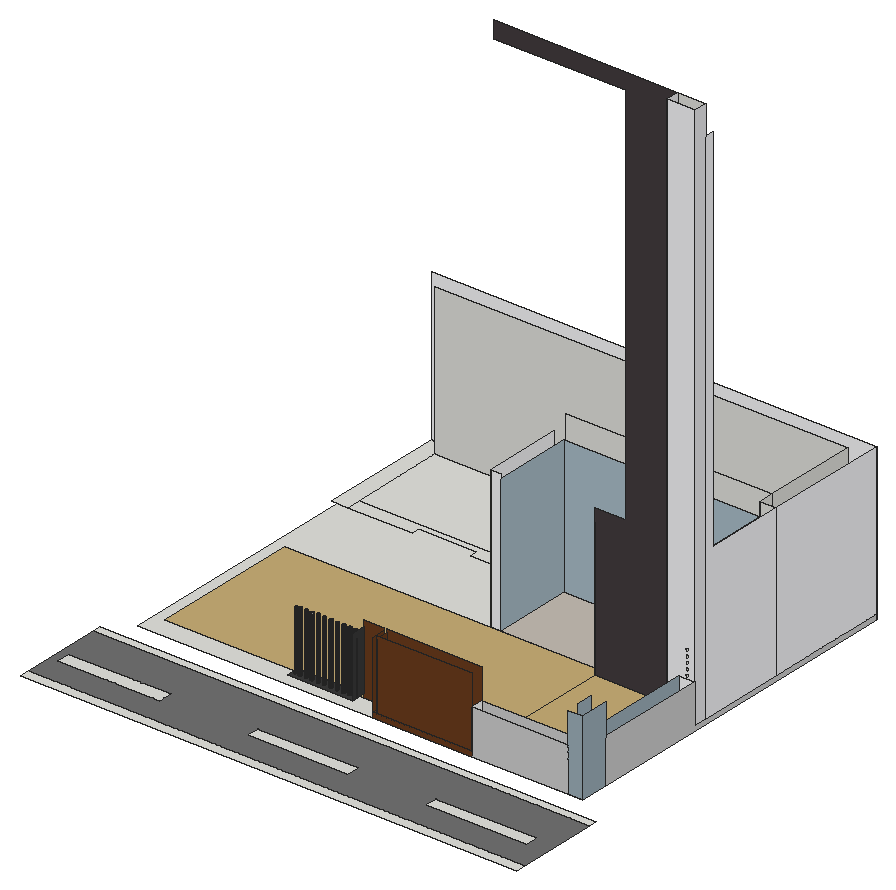
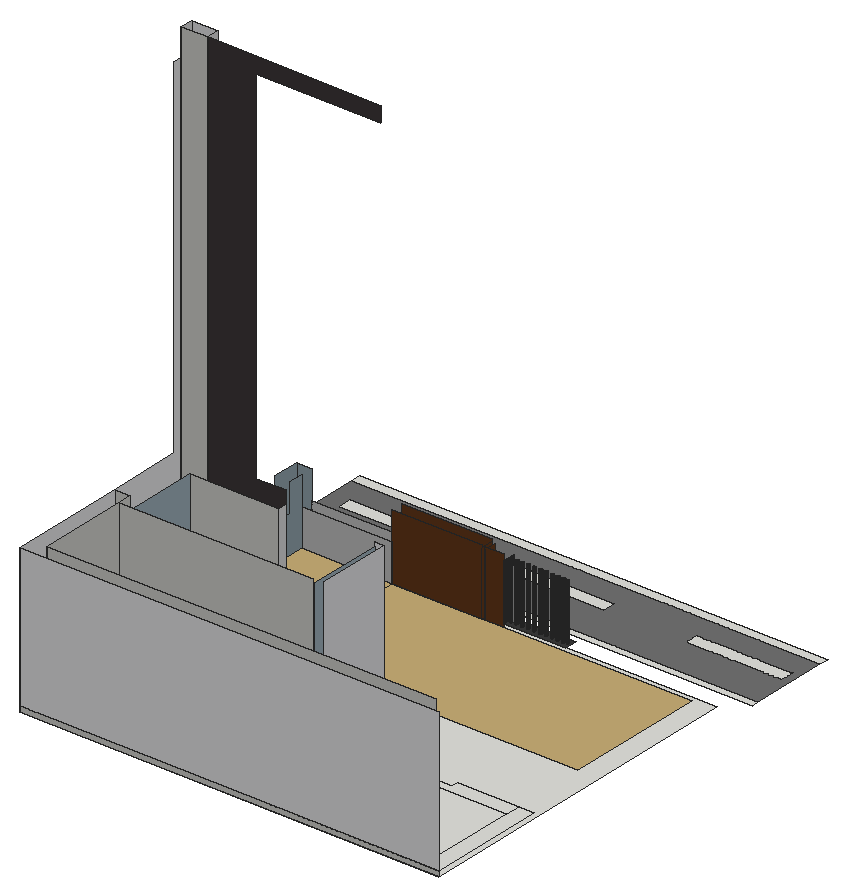
# SketchUp Ruby script. Lengths in inches.
U = 1.inch
M = Sketchup.active_model
def pt(a) = Geom::Point3d.new(a.map { |v| v * U })
def face(e, loops, mat)
  f = e.add_face(loops[0].map { |a| pt(a) })
  loops[1..].each { |l| e.add_face(l.map { |a| pt(a) }).erase! }
  f.material = f.back_material = mat if mat
  f
end
# faces: each face lists its corners as indices into pts; further lists are holes
def faces(e, pts, list, mat = nil) = list.each { |f| face(e, (f[0].is_a?(Array) ? f : [f]).map { |l| l.map { |i| pts[i] } }, mat) }
# xy, xz, yz: faces in a plane at the given z, y or x. An outline is a flat list of corners, or four numbers for a rectangle; further outlines are holes
def ring(l) = l.size == 4 ? [[l[0], l[1]], [l[2], l[1]], [l[2], l[3]], [l[0], l[3]]] : l.each_slice(2).to_a
def flat(e, list, mat, &to3) = list.each { |f| face(e, (f[0].is_a?(Array) ? f : [f]).map { |l| ring(l).map { |u, v| to3.(u, v) } }, mat) }
def xy(e, z, list, mat = nil) = flat(e, list, mat) { |x, y| [x, y, z] }
def xz(e, y, list, mat = nil) = flat(e, list, mat) { |x, z| [x, y, z] }
def yz(e, x, list, mat = nil) = flat(e, list, mat) { |y, z| [x, y, z] }
def lines(e, pts, list) = list.each { |a, b| e.add_line(pt(pts[a]), pt(pts[b])) }
# prism: a flat outline (further loops are holes) pulled along v
def prism(e, loops, v, mat = nil)
  f = face(e, loops, mat); d = Geom::Vector3d.new(v.map { |x| x * U })
  f.pushpull(f.normal.samedirection?(d) ? d.length : -d.length)
end
def box(e, o, s, mat = nil) = prism(e, [[o, [o[0] + s[0], o[1], o[2]], [o[0] + s[0], o[1] + s[1], o[2]], [o[0], o[1] + s[1], o[2]]]], [0, 0, s[2]], mat)
def at(x, y, z, deg = 0) = Geom::Transformation.translation(pt([x, y, z])) * Geom::Transformation.rotation(ORIGIN, Z_AXIS, deg.degrees)
def axes(o, x, y, z) = Geom::Transformation.new([*x, 0, *y, 0, *z, 0, *pt(o).to_a, 1])
def part(name) = M.definitions.add(name)
# library, detail: a bought-in or finely detailed component or shape, given as its bounding box
def library(name, o, s) = part(name).tap { |d| box(d.entities, o, s) }
def detail(e, o, s) = box(e.add_group.entities, o, s)
def put(e, d, t, mat = nil) = e.add_instance(d, t).tap { |i| i.material = mat if mat }
def group(e, t, mat = nil) = e.add_group.tap { |g| g.transformation = t; g.material = mat if mat }.entities
root = M.entities
M.materials.add("[Asphalt New]").color = [67, 60, 62]
M.materials.add("[Blinds Vertical Pattern]").color = [245, 245, 247]
M.materials.add("[Blinds Vertical Pattern]2").color = [234, 234, 237]
M.materials.add("[Blinds Vertical Pattern]3").color = [247, 247, 249]
M.materials.add("[Carrera Marble]").color = [207, 207, 207]
M.materials.add("[Color M03]").color = [170, 170, 170]
M.materials.add("[Color M05]").color = [114, 114, 114]
M.materials.add("[Color M07]").color = [58, 58, 58]
M.materials.add("[Field Rectangle Tile]").color = [196, 189, 179]
M.materials.add("[Formica Speckled Grey]").color = [157, 176, 186]
M.materials.add("[Formica Speckled Grey]2").color = [170, 190, 201]
M.materials.add("[Quartz Light Grey]").color = [251, 251, 252]
M.materials.add("[Tile Limestone Multi]").color = [199, 173, 118]
M.materials.add("[Wood Cherry Original]").color = [107, 60, 29]
xy(root,0,[[0,0,810.125,16.9],[13.43,59.66,179.43,82.41],[321.62,59.66,487.62,82.41],[612.68,59.66,778.68,82.41],[0,150.46,810.125,162.5625],
  [36.42,195.25,761.74,794.75]])
xy(root,0,[[[0,16.9,810.125,150.46],[13.43,59.66,179.43,82.41],[321.62,59.66,487.62,82.41],[612.68,59.66,778.68,82.41]]],"[Color M05]")
xy(root,9,[[425.33,195.25,580.71,216.53],[715.96,423.625,761.74,446.5625],[580.71,446.5625,580.71,461.03,735.46,461.03,735.46,590.55,761.74,590.55,761.74,446.5625],[399.08,461.03,399.08,590.55,262.6,590.55,262.6,602.92,168.16,602.92,168.16,590.55,62.71,590.55,62.71,614.75,735.46,614.75,735.46,590.55,415.32,590.55,415.32,461.03],[36.42,590.55,36.42,794.75,761.74,794.75,761.74,590.55,735.46,590.55,735.46,768.47,62.71,768.47,62.71,590.55],
  [62.71,614.75,735.46,768.47]])
xy(root,9,[[415.32,461.03,735.46,590.55]],"[Field Rectangle Tile]")
xy(root,9,[[62.71,216.53,580.71,461.03],[580.71,216.53,580.71,446.5625,715.96,446.5625,715.96,423.625,736.96,423.625,736.96,216.53]],"[Tile Limestone Multi]")
xy(root,9,[[420.08,195.25,425.33,216.53]],"[Wood Cherry Original]")
xy(root,14.25,[[292.65,202.87,292.05,202.95,291.49,203.18,291.01,203.55,290.64,204.03,290.41,204.58,290.33,205.18,290.41,205.78,290.64,206.34,291.01,206.82,291.49,207.18,292.05,207.42,292.65,207.49,293.24,207.42,293.8,207.18,294.28,206.82,294.65,206.34,294.88,205.78,294.96,205.18,294.88,204.58,294.65,204.03,294.28,203.55,293.8,203.18,293.24,202.95],[302.65,202.87,302.05,202.95,301.49,203.18,301.01,203.55,300.64,204.03,300.41,204.58,300.33,205.18,300.41,205.78,300.64,206.34,301.01,206.82,301.49,207.18,302.05,207.42,302.65,207.49,303.24,207.42,303.8,207.18,304.28,206.82,304.65,206.34,304.88,205.78,304.96,205.18,304.88,204.58,304.65,204.03,304.28,203.55,303.8,203.18,303.24,202.95],[312.15,202.87,311.55,202.95,310.99,203.18,310.51,203.55,310.14,204.03,309.91,204.58,309.83,205.18,309.91,205.78,310.14,206.34,310.51,206.82,310.99,207.18,311.55,207.42,312.15,207.49,312.74,207.42,313.3,207.18,313.78,206.82,314.15,206.34,314.38,205.78,314.46,205.18,314.38,204.58,314.15,204.03,313.78,203.55,313.3,203.18,312.74,202.95],[322.33,202.87,321.73,202.95,321.18,203.18,320.7,203.55,320.33,204.03,320.1,204.58,320.02,205.18,320.1,205.78,320.33,206.34,320.7,206.82,321.18,207.18,321.73,207.42,322.33,207.49,322.93,207.42,323.49,207.18,323.97,206.82,324.34,206.34,324.57,205.78,324.65,205.18,324.57,204.58,324.34,204.03,323.97,203.55,323.49,203.18,322.93,202.95],[332.21,202.87,331.61,202.95,331.05,203.18,330.57,203.55,330.21,204.03,329.97,204.58,329.9,205.18,329.97,205.78,330.21,206.34,330.57,206.82,331.05,207.18,331.61,207.42,332.21,207.49,332.81,207.42,333.36,207.18,333.84,206.82,334.21,206.34,334.44,205.78,334.52,205.18,334.44,204.58,334.21,204.03,333.84,203.55,333.36,203.18,332.81,202.95],
  [343.15,202.87,342.55,202.95,341.99,203.18,341.51,203.55,341.14,204.03,340.91,204.58,340.83,205.18,340.91,205.78,341.14,206.34,341.51,206.82,341.99,207.18,342.55,207.42,343.15,207.49,343.74,207.42,344.3,207.18,344.78,206.82,345.15,206.34,345.38,205.78,345.46,205.18,345.38,204.58,345.15,204.03,344.78,203.55,344.3,203.18,343.74,202.95],[353.71,202.87,353.11,202.95,352.55,203.18,352.07,203.55,351.71,204.03,351.47,204.58,351.4,205.18,351.47,205.78,351.71,206.34,352.07,206.82,352.55,207.18,353.11,207.42,353.71,207.49,354.31,207.42,354.86,207.18,355.34,206.82,355.71,206.34,355.94,205.78,356.02,205.18,355.94,204.58,355.71,204.03,355.34,203.55,354.86,203.18,354.31,202.95],[363.9,202.87,363.3,202.95,362.74,203.18,362.26,203.55,361.89,204.03,361.66,204.58,361.58,205.18,361.66,205.78,361.89,206.34,362.26,206.82,362.74,207.18,363.3,207.42,363.9,207.49,364.49,207.42,365.05,207.18,365.53,206.82,365.9,206.34,366.13,205.78,366.21,205.18,366.13,204.58,365.9,204.03,365.53,203.55,365.05,203.18,364.49,202.95],[373.96,202.87,373.36,202.95,372.8,203.18,372.32,203.55,371.96,204.03,371.72,204.58,371.65,205.18,371.72,205.78,371.96,206.34,372.32,206.82,372.8,207.18,373.36,207.42,373.96,207.49,374.56,207.42,375.11,207.18,375.59,206.82,375.96,206.34,376.19,205.78,376.27,205.18,376.19,204.58,375.96,204.03,375.59,203.55,375.11,203.18,374.56,202.95],[382.71,202.87,382.11,202.95,381.55,203.18,381.07,203.55,380.71,204.03,380.47,204.58,380.4,205.18,380.47,205.78,380.71,206.34,381.07,206.82,381.55,207.18,382.11,207.42,382.71,207.49,383.31,207.42,383.86,207.18,384.34,206.82,384.71,206.34,384.94,205.78,385.02,205.18,384.94,204.58,384.71,204.03,384.34,203.55,383.86,203.18,383.31,202.95]])
xy(root,14.25,[[[280.09,195.25,387.25,216.53],[283.71,202.87,283.11,202.95,282.55,203.18,282.07,203.55,281.71,204.03,281.47,204.58,281.4,205.18,281.47,205.78,281.71,206.34,282.07,206.82,282.55,207.18,283.11,207.42,283.71,207.49,284.31,207.42,284.86,207.18,285.34,206.82,285.71,206.34,285.94,205.78,286.02,205.18,285.94,204.58,285.71,204.03,285.34,203.55,284.86,203.18,284.31,202.95],[292.65,202.87,292.05,202.95,291.49,203.18,291.01,203.55,290.64,204.03,290.41,204.58,290.33,205.18,290.41,205.78,290.64,206.34,291.01,206.82,291.49,207.18,292.05,207.42,292.65,207.49,293.24,207.42,293.8,207.18,294.28,206.82,294.65,206.34,294.88,205.78,294.96,205.18,294.88,204.58,294.65,204.03,294.28,203.55,293.8,203.18,293.24,202.95],[382.71,202.87,382.11,202.95,381.55,203.18,381.07,203.55,380.71,204.03,380.47,204.58,380.4,205.18,380.47,205.78,380.71,206.34,381.07,206.82,381.55,207.18,382.11,207.42,382.71,207.49,383.31,207.42,383.86,207.18,384.34,206.82,384.71,206.34,384.94,205.78,385.02,205.18,384.94,204.58,384.71,204.03,384.34,203.55,383.86,203.18,383.31,202.95],[302.65,202.87,302.05,202.95,301.49,203.18,301.01,203.55,300.64,204.03,300.41,204.58,300.33,205.18,300.41,205.78,300.64,206.34,301.01,206.82,301.49,207.18,302.05,207.42,302.65,207.49,303.24,207.42,303.8,207.18,304.28,206.82,304.65,206.34,304.88,205.78,304.96,205.18,304.88,204.58,304.65,204.03,304.28,203.55,303.8,203.18,303.24,202.95],[373.96,202.87,373.36,202.95,372.8,203.18,372.32,203.55,371.96,204.03,371.72,204.58,371.65,205.18,371.72,205.78,371.96,206.34,372.32,206.82,372.8,207.18,373.36,207.42,373.96,207.49,374.56,207.42,375.11,207.18,375.59,206.82,375.96,206.34,376.19,205.78,376.27,205.18,376.19,204.58,375.96,204.03,375.59,203.55,375.11,203.18,374.56,202.95],[312.15,202.87,311.55,202.95,310.99,203.18,310.51,203.55,310.14,204.03,309.91,204.58,309.83,205.18,309.91,205.78,310.14,206.34,310.51,206.82,310.99,207.18,311.55,207.42,312.15,207.49,312.74,207.42,313.3,207.18,313.78,206.82,314.15,206.34,314.38,205.78,314.46,205.18,314.38,204.58,314.15,204.03,313.78,203.55,313.3,203.18,312.74,202.95],[363.9,202.87,363.3,202.95,362.74,203.18,362.26,203.55,361.89,204.03,361.66,204.58,361.58,205.18,361.66,205.78,361.89,206.34,362.26,206.82,362.74,207.18,363.3,207.42,363.9,207.49,364.49,207.42,365.05,207.18,365.53,206.82,365.9,206.34,366.13,205.78,366.21,205.18,366.13,204.58,365.9,204.03,365.53,203.55,365.05,203.18,364.49,202.95],[322.33,202.87,321.73,202.95,321.18,203.18,320.7,203.55,320.33,204.03,320.1,204.58,320.02,205.18,320.1,205.78,320.33,206.34,320.7,206.82,321.18,207.18,321.73,207.42,322.33,207.49,322.93,207.42,323.49,207.18,323.97,206.82,324.34,206.34,324.57,205.78,324.65,205.18,324.57,204.58,324.34,204.03,323.97,203.55,323.49,203.18,322.93,202.95],[353.71,202.87,353.11,202.95,352.55,203.18,352.07,203.55,351.71,204.03,351.47,204.58,351.4,205.18,351.47,205.78,351.71,206.34,352.07,206.82,352.55,207.18,353.11,207.42,353.71,207.49,354.31,207.42,354.86,207.18,355.34,206.82,355.71,206.34,355.94,205.78,356.02,205.18,355.94,204.58,355.71,204.03,355.34,203.55,354.86,203.18,354.31,202.95],[332.21,202.87,331.61,202.95,331.05,203.18,330.57,203.55,330.21,204.03,329.97,204.58,329.9,205.18,329.97,205.78,330.21,206.34,330.57,206.82,331.05,207.18,331.61,207.42,332.21,207.49,332.81,207.42,333.36,207.18,333.84,206.82,334.21,206.34,334.44,205.78,334.52,205.18,334.44,204.58,334.21,204.03,333.84,203.55,333.36,203.18,332.81,202.95],[343.15,202.87,342.55,202.95,341.99,203.18,341.51,203.55,341.14,204.03,340.91,204.58,340.83,205.18,340.91,205.78,341.14,206.34,341.51,206.82,341.99,207.18,342.55,207.42,343.15,207.49,343.74,207.42,344.3,207.18,344.78,206.82,345.15,206.34,345.38,205.78,345.46,205.18,345.38,204.58,345.15,204.03,344.78,203.55,344.3,203.18,343.74,202.95]]],"[Color M07]")
xz(root,195.25,[[580.71,0,736.96,72.8125]],"[Carrera Marble]")
xz(root,195.25,[[736.96,0,761.74,122.8125]],"[Formica Speckled Grey]")
xz(root,195.25,[[420.08,0,580.71,9],[425.33,9,580.71,122.8125]],"[Wood Cherry Original]")
xz(root,216.53,[[580.71,9,736.96,72.8125]],"[Carrera Marble]")
xz(root,216.53,[[387.25,9,420.08,122.8125],[425.33,9,580.71,122.8125]],"[Wood Cherry Original]")
xz(root,423.625,[[[715.96,9,736.96,9,736.96,72.8125,761.74,72.8125,761.74,908.98,715.96,908.98],[749.95,112.77,749.11,112.88,748.32,113.2,747.65,113.72,747.13,114.39,746.81,115.18,746.7,116.02,746.81,116.86,747.13,117.64,747.65,118.32,748.32,118.83,749.11,119.16,749.95,119.27,750.79,119.16,751.57,118.83,752.24,118.32,752.76,117.64,753.09,116.86,753.2,116.02,753.09,115.18,752.76,114.39,752.24,113.72,751.57,113.2,750.79,112.88],[749.95,102.77,749.11,102.88,748.32,103.2,747.65,103.72,747.13,104.39,746.81,105.18,746.7,106.02,746.81,106.86,747.13,107.64,747.65,108.32,748.32,108.83,749.11,109.16,749.95,109.27,750.79,109.16,751.57,108.83,752.24,108.32,752.76,107.64,753.09,106.86,753.2,106.02,753.09,105.18,752.76,104.39,752.24,103.72,751.57,103.2,750.79,102.88],[749.95,93.33,749.11,93.44,748.32,93.77,747.65,94.28,747.13,94.95,746.81,95.74,746.7,96.58,746.81,97.42,747.13,98.2,747.65,98.88,748.32,99.39,749.11,99.72,749.95,99.83,750.79,99.72,751.57,99.39,752.24,98.88,752.76,98.2,753.09,97.42,753.2,96.58,753.09,95.74,752.76,94.95,752.24,94.28,751.57,93.77,750.79,93.44],[749.95,84.2,749.11,84.32,748.32,84.64,747.65,85.16,747.13,85.83,746.81,86.61,746.7,87.45,746.81,88.3,747.13,89.08,747.65,89.75,748.32,90.27,749.11,90.59,749.95,90.7,750.79,90.59,751.57,90.27,752.24,89.75,752.76,89.08,753.09,88.3,753.2,87.45,753.09,86.61,752.76,85.83,752.24,85.16,751.57,84.64,750.79,84.32],[749.95,74.64,749.11,74.75,748.32,75.08,747.65,75.59,747.13,76.27,746.81,77.05,746.7,77.89,746.81,78.73,747.13,79.52,747.65,80.19,748.32,80.71,749.11,81.03,749.95,81.14,750.79,81.03,751.57,80.71,752.24,80.19,752.76,79.52,753.09,78.73,753.2,77.89,753.09,77.05,752.76,76.27,752.24,75.59,751.57,75.08,750.79,74.75]]],"[Blinds Vertical Pattern]")
xz(root,423.625,[[736.96,9,761.74,72.8125]],"[Quartz Light Grey]")
xz(root,446.5625,[[715.96,9,761.74,908.98]])
xz(root,446.5625,[[580.71,9,715.96,9,715.96,908.98,415.32,908.98,415.32,882.375,631.7,882.375,631.7,254.375,580.71,254.375]],"[Asphalt New]")
xz(root,461.03,[[580.71,9,735.46,231.5625]])
xz(root,461.03,[[399.08,9,415.32,238.875]],"[Blinds Vertical Pattern]")
xz(root,590.55,[[735.46,9,761.74,254.375]])
xz(root,590.55,[[415.32,9,735.46,231.5625]],"[Formica Speckled Grey]2")
xz(root,614.75,[[399.08,9,735.46,254.375]])
xz(root,768.47,[[62.71,9,735.46,254.375]])
xz(root,794.75,[[36.42,0,761.74,9]])
xz(root,794.75,[[36.42,9,761.74,254.375]],"[Blinds Vertical Pattern]3")
yz(root,387.25,[[195.25,14.25,216.53,112.6]],"[Color M07]")
yz(root,399.08,[[461.03,9,590.55,238.875]],"[Blinds Vertical Pattern]")
yz(root,415.32,[[461.03,9,590.55,231.5625]],"[Formica Speckled Grey]2")
yz(root,420.08,[[195.25,9,216.53,117.97]],"[Wood Cherry Original]")
yz(root,425.33,[[195.25,9,216.53,117.97]],"[Wood Cherry Original]")
yz(root,580.71,[[446.5625,9,461.03,231.5625]],"[Blinds Vertical Pattern]2")
yz(root,580.71,[[195.25,9,216.53,72.8125]],"[Quartz Light Grey]")
yz(root,715.96,[[423.625,9,446.5625,908.98]],"[Blinds Vertical Pattern]2")
yz(root,735.46,[[590.55,9,614.75,254.375],[614.75,9,768.47,254.375]])
yz(root,735.46,[[461.03,9,590.55,231.5625]],"[Formica Speckled Grey]2")
yz(root,736.96,[[216.53,9,423.625,9,423.625,72.8125,242.62,72.8125,242.62,122.8125,216.53,122.8125]],"[Formica Speckled Grey]")
yz(root,761.74,[[423.625,9,446.5625,908.98]],"[Blinds Vertical Pattern]2")
yz(root,761.74,[[446.5625,9,590.55,9,590.55,254.375,461.03,254.375,461.03,861.625,446.5625,861.625],[590.55,9,794.75,254.375]],"[Blinds Vertical Pattern]3")
yz(root,761.74,[[242.62,0,794.75,0,794.75,9,423.625,9,423.625,72.8125,242.62,72.8125]],"[Carrera Marble]")
yz(root,761.74,[[195.25,0,242.62,122.8125]],"[Formica Speckled Grey]")
p = [[291.49,203.18,14.25],[292.05,202.95,14.25],[292.05,202.95,112.6],[291.49,203.18,112.6],[292.65,202.87,14.25],[292.65,202.87,112.6],
  [293.24,202.95,14.25],[293.24,202.95,112.6],[293.8,203.18,14.25],[293.8,203.18,112.6],[301.49,203.18,14.25],[302.05,202.95,14.25],
  [302.05,202.95,112.6],[301.49,203.18,112.6],[302.65,202.87,14.25],[302.65,202.87,112.6],[303.24,202.95,14.25],[303.24,202.95,112.6],
  [303.8,203.18,14.25],[303.8,203.18,112.6],[310.99,203.18,14.25],[311.55,202.95,14.25],[311.55,202.95,112.6],[310.99,203.18,112.6],
  [312.15,202.87,14.25],[312.15,202.87,112.6],[312.74,202.95,14.25],[312.74,202.95,112.6],[313.3,203.18,14.25],[313.3,203.18,112.6],
  [321.18,203.18,14.25],[321.73,202.95,14.25],[321.73,202.95,113.625],[321.18,203.18,113.625],[322.33,202.87,14.25],[322.33,202.87,113.625],
  [322.93,202.95,14.25],[322.93,202.95,113.625],[323.49,203.18,14.25],[323.49,203.18,113.625],[331.05,203.18,14.25],[331.61,202.95,14.25],
  [331.61,202.95,112.6],[331.05,203.18,112.6],[332.21,202.87,14.25],[332.21,202.87,112.6],[332.81,202.95,14.25],[332.81,202.95,112.6],
  [333.36,203.18,14.25],[333.36,203.18,112.6],[341.99,203.18,14.25],[342.55,202.95,14.25],[342.55,202.95,112.6],[341.99,203.18,112.6],
  [343.15,202.87,14.25],[343.15,202.87,112.6],[343.74,202.95,14.25],[343.74,202.95,112.6],[344.3,203.18,14.25],[344.3,203.18,112.6],
  [352.55,203.18,14.25],[353.11,202.95,14.25],[353.11,202.95,112.6],[352.55,203.18,112.6],[353.71,202.87,14.25],[353.71,202.87,112.6],
  [354.31,202.95,14.25],[354.31,202.95,112.6],[354.86,203.18,14.25],[354.86,203.18,112.6],[362.74,203.18,14.25],[363.3,202.95,14.25],
  [363.3,202.95,112.6],[362.74,203.18,112.6],[363.9,202.87,14.25],[363.9,202.87,112.6],[364.49,202.95,14.25],[364.49,202.95,112.6],
  [365.05,203.18,14.25],[365.05,203.18,112.6],[372.8,203.18,14.25],[373.36,202.95,14.25],[373.36,202.95,112.6],[372.8,203.18,112.6],
  [373.96,202.87,14.25],[373.96,202.87,112.6],[374.56,202.95,14.25],[374.56,202.95,112.6],[375.11,203.18,14.25],[375.11,203.18,112.6],
  [381.55,203.18,14.25],[382.11,202.95,14.25],[382.11,202.95,112.6],[381.55,203.18,112.6],[382.71,202.87,14.25],[382.71,202.87,112.6],
  [383.31,202.95,14.25],[383.31,202.95,112.6],[383.86,203.18,14.25],[383.86,203.18,112.6],[284.86,203.18,14.25],[285.34,203.55,14.25],
  [285.34,203.55,112.6],[284.86,203.18,112.6],[291.01,203.55,14.25],[291.01,203.55,112.6],[294.28,203.55,14.25],[294.28,203.55,112.6],
  [301.01,203.55,14.25],[301.01,203.55,112.6],[304.28,203.55,14.25],[304.28,203.55,112.6],[310.51,203.55,14.25],[310.51,203.55,112.6],
  [313.78,203.55,14.25],[313.78,203.55,112.6],[320.7,203.55,14.25],[320.7,203.55,113.625],[323.97,203.55,14.25],[323.97,203.55,113.625],
  [330.57,203.55,14.25],[330.57,203.55,112.6],[333.84,203.55,14.25],[333.84,203.55,112.6],[341.51,203.55,14.25],[341.51,203.55,112.6],
  [344.78,203.55,14.25],[344.78,203.55,112.6],[352.07,203.55,14.25],[352.07,203.55,112.6],[355.34,203.55,14.25],[355.34,203.55,112.6],
  [362.26,203.55,14.25],[362.26,203.55,112.6],[365.53,203.55,14.25],[365.53,203.55,112.6],[372.32,203.55,14.25],[372.32,203.55,112.6],
  [375.59,203.55,14.25],[375.59,203.55,112.6],[381.07,203.55,14.25],[381.07,203.55,112.6],[384.34,203.55,14.25],[384.34,203.55,112.6],
  [285.71,204.03,14.25],[285.71,204.03,112.6],[290.64,204.03,14.25],[290.64,204.03,112.6],[294.65,204.03,14.25],[294.65,204.03,112.6],
  [300.64,204.03,14.25],[300.64,204.03,112.6],[304.65,204.03,14.25],[304.65,204.03,112.6],[310.14,204.03,14.25],[310.14,204.03,112.6],
  [314.15,204.03,14.25],[314.15,204.03,112.6],[320.33,204.03,14.25],[320.33,204.03,113.625],[324.34,204.03,14.25],[324.34,204.03,113.625],
  [330.21,204.03,14.25],[330.21,204.03,112.6],[334.21,204.03,14.25],[334.21,204.03,112.6],[341.14,204.03,14.25],[341.14,204.03,112.6],
  [345.15,204.03,14.25],[345.15,204.03,112.6],[351.71,204.03,14.25],[351.71,204.03,112.6],[355.71,204.03,14.25],[355.71,204.03,112.6],
  [361.89,204.03,14.25],[361.89,204.03,112.6],[365.9,204.03,14.25],[365.9,204.03,112.6],[371.96,204.03,14.25],[371.96,204.03,112.6],
  [375.96,204.03,14.25],[375.96,204.03,112.6],[380.71,204.03,14.25],[380.71,204.03,112.6],[384.71,204.03,14.25],[384.71,204.03,112.6],
  [285.94,204.58,14.25],[285.94,204.58,112.6],[290.41,204.58,14.25],[290.41,204.58,112.6],[294.88,204.58,14.25],[294.88,204.58,112.6],
  [300.41,204.58,14.25],[300.41,204.58,112.6],[304.88,204.58,14.25],[304.88,204.58,112.6],[309.91,204.58,14.25],[309.91,204.58,112.6],
  [314.38,204.58,14.25],[314.38,204.58,112.6],[320.1,204.58,14.25],[320.1,204.58,113.625],[324.57,204.58,14.25],[324.57,204.58,113.625],
  [329.97,204.58,14.25],[329.97,204.58,112.6],[334.44,204.58,14.25],[334.44,204.58,112.6],[340.91,204.58,14.25],[340.91,204.58,112.6],
  [345.38,204.58,14.25],[345.38,204.58,112.6],[351.47,204.58,14.25],[351.47,204.58,112.6],[355.94,204.58,14.25],[355.94,204.58,112.6],
  [361.66,204.58,14.25],[361.66,204.58,112.6],[366.13,204.58,14.25],[366.13,204.58,112.6],[371.72,204.58,14.25],[371.72,204.58,112.6],
  [376.19,204.58,14.25],[376.19,204.58,112.6],[380.47,204.58,14.25],[380.47,204.58,112.6],[384.94,204.58,14.25],[384.94,204.58,112.6],
  [286.02,205.18,14.25],[286.02,205.18,112.6],[290.33,205.18,14.25],[290.33,205.18,112.6],[294.96,205.18,14.25],[294.96,205.18,112.6],
  [300.33,205.18,14.25],[300.33,205.18,112.6],[304.96,205.18,14.25],[304.96,205.18,112.6],[309.83,205.18,14.25],[309.83,205.18,112.6],
  [314.46,205.18,14.25],[314.46,205.18,112.6],[320.02,205.18,14.25],[320.02,205.18,113.625],[324.65,205.18,14.25],[324.65,205.18,113.625],
  [329.9,205.18,14.25],[329.9,205.18,112.6],[334.52,205.18,14.25],[334.52,205.18,112.6],[340.83,205.18,14.25],[340.83,205.18,112.6],
  [345.46,205.18,14.25],[345.46,205.18,112.6],[351.4,205.18,14.25],[351.4,205.18,112.6],[356.02,205.18,14.25],[356.02,205.18,112.6],
  [361.58,205.18,14.25],[361.58,205.18,112.6],[366.21,205.18,14.25],[366.21,205.18,112.6],[371.65,205.18,14.25],[371.65,205.18,112.6],
  [376.27,205.18,14.25],[376.27,205.18,112.6],[380.4,205.18,14.25],[380.4,205.18,112.6],[385.02,205.18,14.25],[385.02,205.18,112.6],
  [285.94,205.78,14.25],[285.94,205.78,112.6],[290.41,205.78,14.25],[290.41,205.78,112.6],[294.88,205.78,14.25],[294.88,205.78,112.6],
  [300.41,205.78,14.25],[300.41,205.78,112.6],[304.88,205.78,14.25],[304.88,205.78,112.6],[309.91,205.78,14.25],[309.91,205.78,112.6],
  [314.38,205.78,14.25],[314.38,205.78,112.6],[320.1,205.78,14.25],[320.1,205.78,113.625],[324.57,205.78,14.25],[324.57,205.78,113.625],
  [329.97,205.78,14.25],[329.97,205.78,112.6],[334.44,205.78,14.25],[334.44,205.78,112.6],[340.91,205.78,14.25],[340.91,205.78,112.6],
  [345.38,205.78,14.25],[345.38,205.78,112.6],[351.47,205.78,14.25],[351.47,205.78,112.6],[355.94,205.78,14.25],[355.94,205.78,112.6],
  [361.66,205.78,14.25],[361.66,205.78,112.6],[366.13,205.78,14.25],[366.13,205.78,112.6],[371.72,205.78,14.25],[371.72,205.78,112.6],
  [376.19,205.78,14.25],[376.19,205.78,112.6],[380.47,205.78,14.25],[380.47,205.78,112.6],[384.94,205.78,14.25],[384.94,205.78,112.6],
  [285.71,206.34,14.25],[285.71,206.34,112.6],[290.64,206.34,14.25],[290.64,206.34,112.6],[294.65,206.34,14.25],[294.65,206.34,112.6],
  [300.64,206.34,14.25],[300.64,206.34,112.6],[304.65,206.34,14.25],[304.65,206.34,112.6],[310.14,206.34,14.25],[310.14,206.34,112.6],
  [314.15,206.34,14.25],[314.15,206.34,112.6],[320.33,206.34,14.25],[320.33,206.34,113.625],[324.34,206.34,14.25],[324.34,206.34,113.625],
  [330.21,206.34,14.25],[330.21,206.34,112.6],[334.21,206.34,14.25],[334.21,206.34,112.6],[341.14,206.34,14.25],[341.14,206.34,112.6],
  [345.15,206.34,14.25],[345.15,206.34,112.6],[351.71,206.34,14.25],[351.71,206.34,112.6],[355.71,206.34,14.25],[355.71,206.34,112.6],
  [361.89,206.34,14.25],[361.89,206.34,112.6],[365.9,206.34,14.25],[365.9,206.34,112.6],[371.96,206.34,14.25],[371.96,206.34,112.6],
  [375.96,206.34,14.25],[375.96,206.34,112.6],[380.71,206.34,14.25],[380.71,206.34,112.6],[384.71,206.34,14.25],[384.71,206.34,112.6],
  [285.34,206.82,14.25],[285.34,206.82,112.6],[291.01,206.82,14.25],[291.01,206.82,112.6],[294.28,206.82,14.25],[294.28,206.82,112.6],
  [301.01,206.82,14.25],[301.01,206.82,112.6],[304.28,206.82,14.25],[304.28,206.82,112.6],[310.51,206.82,14.25],[310.51,206.82,112.6],
  [313.78,206.82,14.25],[313.78,206.82,112.6],[320.7,206.82,14.25],[320.7,206.82,113.625],[323.97,206.82,14.25],[323.97,206.82,113.625],
  [330.57,206.82,14.25],[330.57,206.82,112.6],[333.84,206.82,14.25],[333.84,206.82,112.6],[341.51,206.82,14.25],[341.51,206.82,112.6],
  [344.78,206.82,14.25],[344.78,206.82,112.6],[352.07,206.82,14.25],[352.07,206.82,112.6],[355.34,206.82,14.25],[355.34,206.82,112.6],
  [362.26,206.82,14.25],[362.26,206.82,112.6],[365.53,206.82,14.25],[365.53,206.82,112.6],[372.32,206.82,14.25],[372.32,206.82,112.6],
  [375.59,206.82,14.25],[375.59,206.82,112.6],[381.07,206.82,14.25],[381.07,206.82,112.6],[384.34,206.82,14.25],[384.34,206.82,112.6],
  [291.49,207.18,14.25],[291.49,207.18,112.6],[293.8,207.18,14.25],[293.8,207.18,112.6],[301.49,207.18,14.25],[301.49,207.18,112.6],
  [303.8,207.18,14.25],[303.8,207.18,112.6],[310.99,207.18,14.25],[310.99,207.18,112.6],[313.3,207.18,14.25],[313.3,207.18,112.6],
  [321.18,207.18,14.25],[321.18,207.18,113.625],[323.49,207.18,14.25],[323.49,207.18,113.625],[331.05,207.18,14.25],[331.05,207.18,112.6],
  [333.36,207.18,14.25],[333.36,207.18,112.6],[341.99,207.18,14.25],[341.99,207.18,112.6],[344.3,207.18,14.25],[344.3,207.18,112.6],
  [352.55,207.18,14.25],[352.55,207.18,112.6],[354.86,207.18,14.25],[354.86,207.18,112.6],[362.74,207.18,14.25],[362.74,207.18,112.6],
  [365.05,207.18,14.25],[365.05,207.18,112.6],[372.8,207.18,14.25],[372.8,207.18,112.6],[375.11,207.18,14.25],[375.11,207.18,112.6],
  [381.55,207.18,14.25],[381.55,207.18,112.6],[383.86,207.18,14.25],[383.86,207.18,112.6],[292.05,207.42,14.25],[292.05,207.42,112.6],
  [293.24,207.42,14.25],[293.24,207.42,112.6],[302.05,207.42,14.25],[302.05,207.42,112.6],[303.24,207.42,14.25],[303.24,207.42,112.6],
  [311.55,207.42,14.25],[311.55,207.42,112.6],[312.74,207.42,14.25],[312.74,207.42,112.6],[321.73,207.42,14.25],[321.73,207.42,113.625],
  [322.93,207.42,14.25],[322.93,207.42,113.625],[331.61,207.42,14.25],[331.61,207.42,112.6],[332.81,207.42,14.25],[332.81,207.42,112.6],
  [342.55,207.42,14.25],[342.55,207.42,112.6],[343.74,207.42,14.25],[343.74,207.42,112.6],[353.11,207.42,14.25],[353.11,207.42,112.6],
  [354.31,207.42,14.25],[354.31,207.42,112.6],[363.3,207.42,14.25],[363.3,207.42,112.6],[364.49,207.42,14.25],[364.49,207.42,112.6],
  [373.36,207.42,14.25],[373.36,207.42,112.6],[374.56,207.42,14.25],[374.56,207.42,112.6],[382.11,207.42,14.25],[382.11,207.42,112.6],
  [383.31,207.42,14.25],[383.31,207.42,112.6],[292.65,207.49,14.25],[292.65,207.49,112.6],[302.65,207.49,14.25],[302.65,207.49,112.6],
  [312.15,207.49,14.25],[312.15,207.49,112.6],[322.33,207.49,14.25],[322.33,207.49,113.625],[332.21,207.49,14.25],[332.21,207.49,112.6],
  [343.15,207.49,14.25],[343.15,207.49,112.6],[353.71,207.49,14.25],[353.71,207.49,112.6],[363.9,207.49,14.25],[363.9,207.49,112.6],
  [373.96,207.49,14.25],[373.96,207.49,112.6],[382.71,207.49,14.25],[382.71,207.49,112.6],[399.08,614.75,0],[399.08,614.75,9]]
faces(root,p,[[0,1,2,3],[1,4,5,2],[4,6,7,5],[6,8,9,7],[10,11,12,13],[11,14,15,12],[14,16,17,15],[16,18,19,17],
  [20,21,22,23],[21,24,25,22],[24,26,27,25],[26,28,29,27],[30,31,32,33],[31,34,35,32],[34,36,37,35],[36,38,39,37],
  [40,41,42,43],[41,44,45,42],[44,46,47,45],[46,48,49,47],[50,51,52,53],[51,54,55,52],[54,56,57,55],[56,58,59,57],
  [60,61,62,63],[61,64,65,62],[64,66,67,65],[66,68,69,67],[70,71,72,73],[71,74,75,72],[74,76,77,75],[76,78,79,77],
  [80,81,82,83],[81,84,85,82],[84,86,87,85],[86,88,89,87],[90,91,92,93],[91,94,95,92],[94,96,97,95],[96,98,99,97],
  [100,101,102,103],[104,0,3,105],[8,106,107,9],[108,10,13,109],[18,110,111,19],[112,20,23,113],[28,114,115,29],[116,30,33,117],
  [38,118,119,39],[120,40,43,121],[48,122,123,49],[124,50,53,125],[58,126,127,59],[128,60,63,129],[68,130,131,69],[132,70,73,133],
  [78,134,135,79],[136,80,83,137],[88,138,139,89],[140,90,93,141],[98,142,143,99],[101,144,145,102],[146,104,105,147],[106,148,149,107],
  [150,108,109,151],[110,152,153,111],[154,112,113,155],[114,156,157,115],[158,116,117,159],[118,160,161,119],[162,120,121,163],[122,164,165,123],
  [166,124,125,167],[126,168,169,127],[170,128,129,171],[130,172,173,131],[174,132,133,175],[134,176,177,135],[178,136,137,179],[138,180,181,139],
  [182,140,141,183],[142,184,185,143],[144,186,187,145],[188,146,147,189],[148,190,191,149],[192,150,151,193],[152,194,195,153],[196,154,155,197],
  [156,198,199,157],[200,158,159,201],[160,202,203,161],[204,162,163,205],[164,206,207,165],[208,166,167,209],[168,210,211,169],[212,170,171,213],
  [172,214,215,173],[216,174,175,217],[176,218,219,177],[220,178,179,221],[180,222,223,181],[224,182,183,225],[184,226,227,185],[186,228,229,187],
  [230,188,189,231],[190,232,233,191],[234,192,193,235],[194,236,237,195],[238,196,197,239],[198,240,241,199],[242,200,201,243],[202,244,245,203],
  [246,204,205,247],[206,248,249,207],[250,208,209,251],[210,252,253,211],[254,212,213,255],[214,256,257,215],[258,216,217,259],[218,260,261,219],
  [262,220,221,263],[222,264,265,223],[266,224,225,267],[226,268,269,227],[228,270,271,229],[272,230,231,273],[232,274,275,233],[276,234,235,277],
  [236,278,279,237],[280,238,239,281],[240,282,283,241],[284,242,243,285],[244,286,287,245],[288,246,247,289],[248,290,291,249],[292,250,251,293],
  [252,294,295,253],[296,254,255,297],[256,298,299,257],[300,258,259,301],[260,302,303,261],[304,262,263,305],[264,306,307,265],[308,266,267,309],
  [268,310,311,269],[270,312,313,271],[314,272,273,315],[274,316,317,275],[318,276,277,319],[278,320,321,279],[322,280,281,323],[282,324,325,283],
  [326,284,285,327],[286,328,329,287],[330,288,289,331],[290,332,333,291],[334,292,293,335],[294,336,337,295],[338,296,297,339],[298,340,341,299],
  [342,300,301,343],[302,344,345,303],[346,304,305,347],[306,348,349,307],[350,308,309,351],[310,352,353,311],[312,354,355,313],[356,314,315,357],
  [316,358,359,317],[360,318,319,361],[320,362,363,321],[364,322,323,365],[324,366,367,325],[368,326,327,369],[328,370,371,329],[372,330,331,373],
  [332,374,375,333],[376,334,335,377],[336,378,379,337],[380,338,339,381],[340,382,383,341],[384,342,343,385],[344,386,387,345],[388,346,347,389],
  [348,390,391,349],[392,350,351,393],[352,394,395,353],[396,356,357,397],[358,398,399,359],[400,360,361,401],[362,402,403,363],[404,364,365,405],
  [366,406,407,367],[408,368,369,409],[370,410,411,371],[412,372,373,413],[374,414,415,375],[416,376,377,417],[378,418,419,379],[420,380,381,421],
  [382,422,423,383],[424,384,385,425],[386,426,427,387],[428,388,389,429],[390,430,431,391],[432,392,393,433],[394,434,435,395],[436,396,397,437],
  [398,438,439,399],[440,400,401,441],[402,442,443,403],[444,404,405,445],[406,446,447,407],[448,408,409,449],[410,450,451,411],[452,412,413,453],
  [414,454,455,415],[456,416,417,457],[418,458,459,419],[460,420,421,461],[422,462,463,423],[464,424,425,465],[426,466,467,427],[468,428,429,469],
  [430,470,471,431],[472,432,433,473],[434,474,475,435],[476,436,437,477],[438,476,477,439],[478,440,441,479],[442,478,479,443],[480,444,445,481],
  [446,480,481,447],[482,448,449,483],[450,482,483,451],[484,452,453,485],[454,484,485,455],[486,456,457,487],[458,486,487,459],[488,460,461,489],
  [462,488,489,463],[490,464,465,491],[466,490,491,467],[492,468,469,493],[470,492,493,471],[494,472,473,495],[474,494,495,475]],"[Color M03]")
lines(root,p,[[496,497]])
